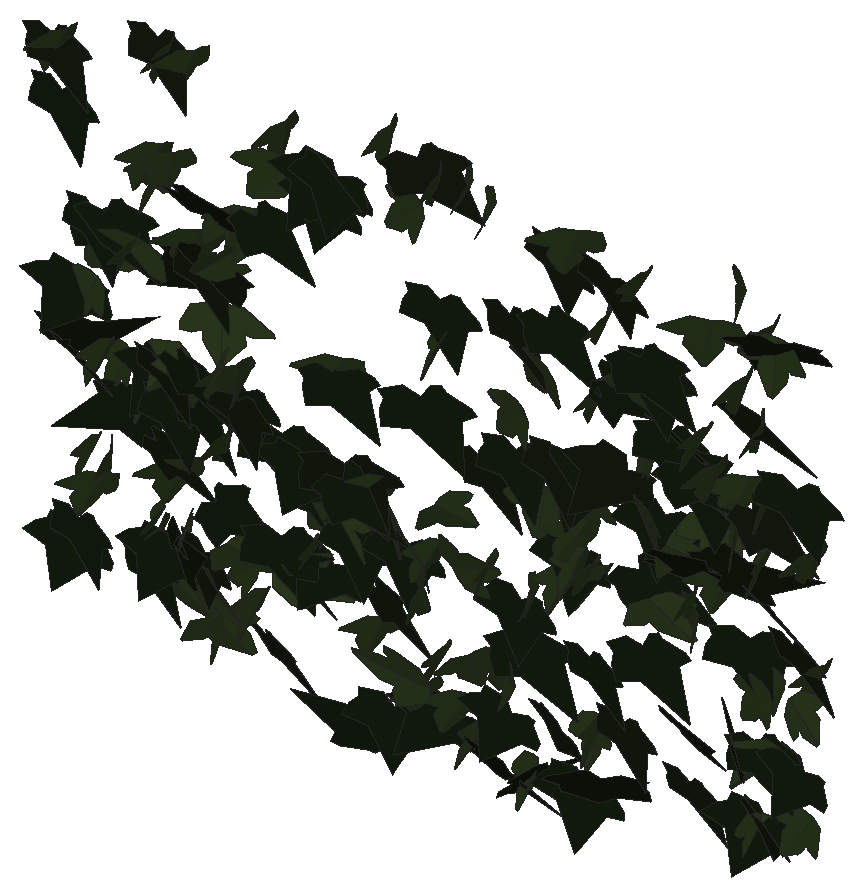
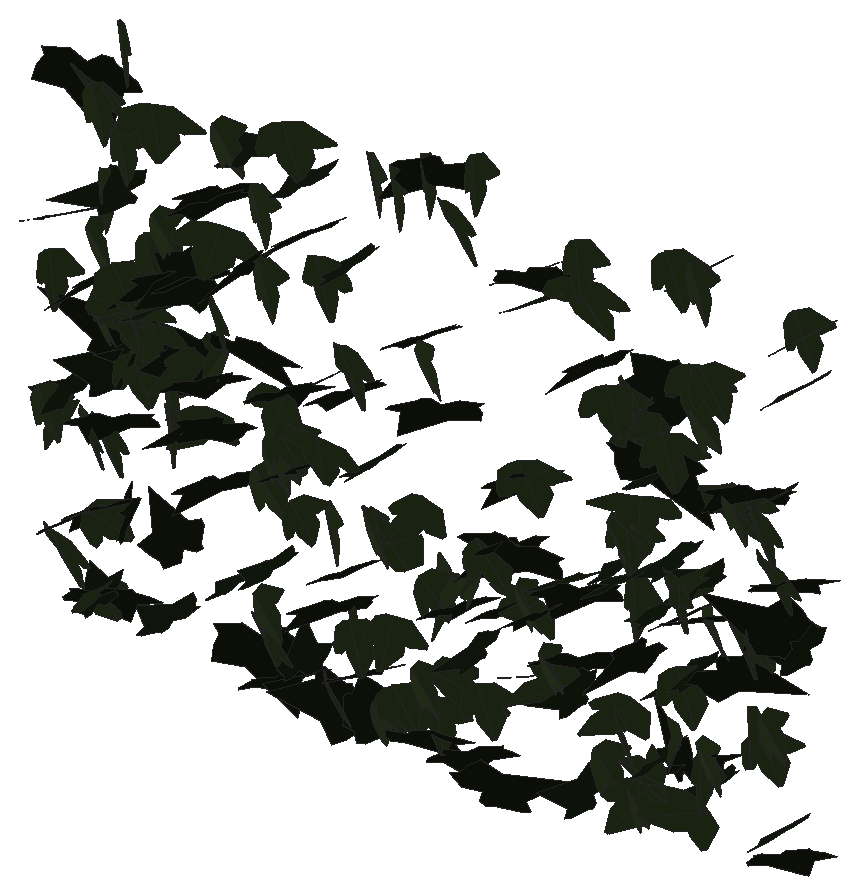
# SketchUp Ruby script. Lengths in millimetres.
U = 1.mm
M = Sketchup.active_model
def pt(a) = Geom::Point3d.new(a.map { |v| v * U })
def face(e, loops, mat)
  f = e.add_face(loops[0].map { |a| pt(a) })
  loops[1..].each { |l| e.add_face(l.map { |a| pt(a) }).erase! }
  f.material = f.back_material = mat if mat
  f
end
# faces: each face lists its corners as indices into pts; further lists are holes
def faces(e, pts, list, mat = nil) = list.each { |f| face(e, (f[0].is_a?(Array) ? f : [f]).map { |l| l.map { |i| pts[i] } }, mat) }
# xy, xz, yz: faces in a plane at the given z, y or x. An outline is a flat list of corners, or four numbers for a rectangle; further outlines are holes
def ring(l) = l.size == 4 ? [[l[0], l[1]], [l[2], l[1]], [l[2], l[3]], [l[0], l[3]]] : l.each_slice(2).to_a
def flat(e, list, mat, &to3) = list.each { |f| face(e, (f[0].is_a?(Array) ? f : [f]).map { |l| ring(l).map { |u, v| to3.(u, v) } }, mat) }
def xy(e, z, list, mat = nil) = flat(e, list, mat) { |x, y| [x, y, z] }
def xz(e, y, list, mat = nil) = flat(e, list, mat) { |x, z| [x, y, z] }
def yz(e, x, list, mat = nil) = flat(e, list, mat) { |y, z| [x, y, z] }
def lines(e, pts, list) = list.each { |a, b| e.add_line(pt(pts[a]), pt(pts[b])) }
# prism: a flat outline (further loops are holes) pulled along v
def prism(e, loops, v, mat = nil)
  f = face(e, loops, mat); d = Geom::Vector3d.new(v.map { |x| x * U })
  f.pushpull(f.normal.samedirection?(d) ? d.length : -d.length)
end
def box(e, o, s, mat = nil) = prism(e, [[o, [o[0] + s[0], o[1], o[2]], [o[0] + s[0], o[1] + s[1], o[2]], [o[0], o[1] + s[1], o[2]]]], [0, 0, s[2]], mat)
def at(x, y, z, deg = 0) = Geom::Transformation.translation(pt([x, y, z])) * Geom::Transformation.rotation(ORIGIN, Z_AXIS, deg.degrees)
def axes(o, x, y, z) = Geom::Transformation.new([*x, 0, *y, 0, *z, 0, *pt(o).to_a, 1])
def part(name) = M.definitions.add(name)
# library, detail: a bought-in or finely detailed component or shape, given as its bounding box
def library(name, o, s) = part(name).tap { |d| box(d.entities, o, s) }
def detail(e, o, s) = box(e.add_group.entities, o, s)
def put(e, d, t, mat = nil) = e.add_instance(d, t).tap { |i| i.material = mat if mat }
def group(e, t, mat = nil) = e.add_group.tap { |g| g.transformation = t; g.material = mat if mat }.entities
root = M.entities
M.materials.add("efeu1").color = [18, 25, 13]
M.materials.add("efeu2").color = [43, 57, 29]
c1 = part("ivyleaf_9")
p = [[39.1,54.8,31.7],[34.5,51.8,30.2],[-5.3,25.2,17.3],[-17.9,28.3,20.9],[-21.6,21.7,17],[-20.2,4.3,5.3],
  [-22.9,-0.3,2.5],[-17.1,-4,-0.6],[-2,-2.1,-1.2],[-0.7,-15.4,-10.1],[16.6,-22.3,-16.7],[21.1,-15.1,-12.5],
  [32.7,-10.7,-11],[46.1,-1.8,-6.6],[30.8,11.2,3.8]]
faces(c1.entities,p,[[0,1,2,3,4,5,6,7,8,9,10,11,12,13,14]],"efeu1")
c2 = part("ivyleaf_10")
p = [[0,12.8,-0.8],[-1.5,51.3,-10.9],[-4.9,51,-11.6],[-13.6,26.5,-7.3],[-13.2,15.9,-4.6],[-21.1,19.3,-7.2],
  [-29.5,16.3,-8.3],[-29.2,8.3,-6.2],[-19.7,-9.8,0.5],[-7.6,-13,4],[1,-12.2,5.8],[-0.4,51.1,-11.1],
  [-1.5,51.1,-10.9],[1,-12.4,5.9],[16.9,-12.4,3.5],[35.1,9.1,-5.1],[35,12.9,-6.1],[20.5,16.4,-4.9],
  [15.8,15,-3.8],[15.3,27.6,-7.1],[12.8,31.3,-7.8]]
faces(c2.entities,p,[[0,1,2,3,4,5,6,7,8,9,10],[11,12,0,13,14,15,16,17,18,19,20]],"efeu2")
put(root,c1,axes([2801.1,826.6,2664.1],[-1.10955,-0.82912,0.08509],[-0.11702,-0.06078,-1.01345],[1.58194,-0.58603,-0.01529]))
put(root,c2,axes([2807.7,780.4,3394.3],[-0.3467,-1.12207,0.06098],[-0.01451,-0.06054,-1.13675],[2.13862,-0.18231,0.00218]))
put(root,c1,axes([2775.7,808.9,2958],[1.15219,-0.84979,0.25487],[0.27577,-0.2097,-1.04338],[1.66582,0.62248,-0.00356]))
put(root,c1,axes([2816.9,808,3034.7],[-1.24222,-0.80833,0.30515],[-0.17317,-0.316,-1.0317],[1.63524,-0.64752,0.12255]))
put(root,c1,axes([2794,785.9,3384.4],[0.30526,-1.10682,-0.1239],[-0.02359,0.1234,-1.11837],[2.11953,0.16078,0.0054]))
put(root,c1,axes([2803.6,791.1,3306.8],[0.05728,-1.13304,0.14401],[-0.01395,-0.14425,-1.13339],[2.1737,0.02893,-0.01107]))
put(root,c1,axes([2806.6,820.6,2691.5],[0.14849,-1.05092,0.15369],[-0.03699,-0.15549,-1.05337],[2.02105,0.07437,-0.03057]))
put(root,c2,axes([2836.9,800.2,3044.7],[1.54076,-0.74256,-0.07024],[-0.09909,0.04716,-1.09854],[1.41609,0.81123,-0.00044]))
put(root,c2,axes([2840.7,803.3,2821.8],[0.26864,-1.00933,0.37026],[0.19743,-0.35891,-1.01793],[2.03658,0.16793,0.04984]))
put(root,c1,axes([2812,803,2958],[0.25424,-0.24109,1.08514],[2.02552,0.34325,-0.05475],[-0.61074,1.03805,0.27013]))
put(root,c2,axes([2849,811.8,3116.8],[1.37351,-0.76625,-0.26758],[-0.18364,0.27452,-1.04638],[1.53374,0.71907,0.11434]))
put(root,c2,axes([2848.9,815.4,2954.1],[-0.04483,-1.01285,0.35435],[0.15288,-0.3551,-1.00967],[2.03649,0.00436,0.08359]))
put(root,c2,axes([2861.5,786.7,2782.8],[-0.75736,-0.95193,0.27209],[-0.06897,-0.27905,-1.02926],[1.88301,-0.3931,0.07174]))
put(root,c1,axes([2843.6,807.7,3140.8],[0.01858,-1.10197,0.19045],[0.00835,-0.19042,-1.10201],[2.12835,0.01036,0.00266]))
put(root,c2,axes([2870.9,797,2819.4],[0.28302,-0.96486,-0.42015],[0.12334,0.43191,-0.96894],[1.99907,0.10995,0.11927]))
put(root,c2,axes([2874.8,818.4,2947.8],[1.28393,-0.84668,-0.05431],[-0.05125,0.04798,-1.08254],[1.6139,0.6751,0.00883]))
put(root,c1,axes([2900.1,820.3,2888.5],[-0.06741,-0.21643,-1.12372],[-0.26118,-1.11534,0.21915],[-2.16226,0.14147,0.00856]))
put(root,c1,axes([2862.3,805.3,3149],[-0.06879,-0.87646,-0.66877],[0.48857,0.64404,-0.85793],[2.04053,-0.18375,0.18287]))
put(root,c2,axes([2907.8,797.3,3122.4],[1.76347,0.1574,-0.59669],[-1.17438,0.22347,-0.89926],[-0.01402,1.07919,0.27324]))
put(root,c2,axes([2900.4,802.6,3121.8],[0.24739,-1.08128,0.03849],[-0.02294,-0.04022,-1.08894],[2.05907,0.12946,-0.01675]))
put(root,c2,axes([2925.9,808.6,2936],[1.02094,-0.86378,0.36948],[0.3238,-0.32912,-1.01643],[1.75847,0.5621,-0.02735]))
put(root,c2,axes([2937.8,807.8,2752.4],[0.47727,-1.00004,0.05704],[-0.01289,-0.06049,-1.03078],[1.90632,0.24996,-0.02125]))
put(root,c2,axes([2936.1,819,3229.4],[0.33367,-0.94598,0.53413],[0.22354,-0.52136,-0.96192],[2.05542,0.21027,0.01791]))
put(root,c2,axes([2941.3,805.3,2732.3],[-0.08638,-0.98582,-0.46393],[0.13683,0.46061,-0.9858],[2.06906,-0.07162,0.04582]))
put(root,c2,axes([2945.3,793.7,3273.5],[-0.45942,-1.07051,0.30346],[-0.00104,-0.31041,-1.09545],[2.11768,-0.2324,0.0653]))
put(root,c1,axes([2945.8,825.3,2946.2],[-1.22139,-0.75796,0.41022],[-0.15538,-0.4557,-0.9697],[1.63289,-0.61031,0.21457]))
put(root,c2,axes([2956.4,800.5,3417.3],[0.14916,-1.1181,-0.11985],[0.03099,0.12126,-1.12057],[2.13993,0.07618,0.02458]))
put(root,c1,axes([2936.6,792,2697.5],[0.47251,-1.02616,0.13462],[0.05397,-0.13165,-1.05576],[1.96897,0.24986,-0.00337]))
put(root,c2,axes([2967.1,794.3,3269.1],[-0.98097,-1.00778,-0.09552],[0.0936,0.08214,-1.13192],[1.92432,-0.51773,0.00636]))
put(root,c1,axes([2948.2,799.4,3427.7],[0.1969,-1.12618,-0.01265],[-0.00764,0.01234,-1.13092],[2.14346,0.1035,-0.00287]))
put(root,c2,axes([2968.2,812.2,2978],[-0.49162,-0.3332,1.00297],[0.29915,-1.03312,-0.30273],[1.98906,0.07303,0.29343]))
put(root,c1,axes([2970.3,792.8,2720.7],[-0.95462,-0.87184,0.30464],[-0.26067,-0.27262,-1.00569],[1.73823,-0.51969,0.01649]))
put(root,c2,axes([2979.8,799.7,2837.4],[-0.88497,-1.06092,0.0823],[-0.029,-0.08316,-1.15818],[2.025,-0.46483,0.01938]))
put(root,c1,axes([2951.6,797.1,2860.4],[1.22153,-0.75905,-0.41264],[-0.26761,0.41541,-0.98287],[1.62236,0.64004,0.14856]))
put(root,c2,axes([2950.3,815.2,2668.4],[-1.41336,0.26915,-0.83997],[1.51063,-0.27496,-0.78985],[-0.73213,-1.08694,-0.00819]))
put(root,c2,axes([2993.8,793.4,2742.7],[0.10618,-0.03913,1.05907],[-0.9757,0.9272,0.06126],[-1.76531,-0.51482,0.02984]))
put(root,c1,axes([2959.6,793.7,2972.2],[0.18973,-0.9481,0.51024],[0.33745,-0.49097,-0.94694],[2.02117,0.17097,0.1102]))
put(root,c2,axes([2992.5,802.7,2972.6],[1.16461,-0.80627,-0.41024],[-0.25459,0.40919,-1.00374],[1.70278,0.61263,0.13051]))
put(root,c2,axes([2995.5,800.6,3421.7],[-0.60731,-1.08053,0.06525],[-0.01505,-0.0657,-1.12661],[2.06015,-0.31901,0.01101]))
put(root,c2,axes([2997.4,808.2,3166.3],[-0.98211,-0.96649,0.0334],[-0.0227,-0.0315,-1.09562],[1.84039,-0.51615,0.00431]))
put(root,c1,axes([2978.2,793,2928.8],[-0.09021,-1.08135,0.06935],[0.01532,-0.06976,-1.08233],[2.0622,-0.04678,0.01108]))
put(root,c1,axes([3027.8,798.5,3141.1],[0.73257,0.23675,-1.07574],[-1.69913,-0.60038,-0.45158],[-1.22786,0.97207,-0.01691]))
put(root,c1,axes([2984.2,794.1,2711.9],[-0.03752,0.14168,1.08472],[0.32188,-1.07146,0.14302],[2.05694,0.17025,-0.00259]))
put(root,c1,axes([2996,783.1,2996.1],[1.01436,-0.92924,-0.2297],[-0.06113,0.2454,-1.06727],[1.82073,0.52593,0.09214]))
put(root,c1,axes([3008.2,814.4,2716.8],[-0.04258,-0.91012,0.53359],[-0.05345,-0.53301,-0.91031],[2.00719,-0.0335,-0.01292]))
put(root,c1,axes([2999.2,806,2935.1],[0.65484,-1.06382,-0.00474],[-0.00264,0.00453,-1.11808],[2.02468,0.34407,0.00007]))
put(root,c1,axes([3009.8,807.8,3123.6],[0.16596,-1.02644,0.33344],[0.24682,-0.32214,-1.02556],[2.03913,0.12253,0.097]))
put(root,c1,axes([3002.1,783.3,3233.9],[2.01866,-0.29857,0.25163],[0.46138,-0.06743,-1.10189],[0.58255,1.08802,0.00076]))
put(root,c2,axes([3040.1,779,3188.3],[-0.03065,-0.263,-1.09291],[0.38139,1.07484,-0.2616],[2.10514,-0.19856,0.03148]))
put(root,c2,axes([3015.1,803.6,2684.5],[0.2018,-0.24599,1.06458],[1.86659,-0.45001,-0.20167],[0.91657,0.9706,0.1763]))
put(root,c2,axes([3041,804.7,3069],[1.74046,0.73038,-0.01547],[-0.0229,-0.00973,-1.17036],[-1.39019,0.91457,-0.00009]))
put(root,c2,axes([3049.4,803.1,2646.5],[0.40297,-0.93259,0.56746],[0.48337,-0.52009,-0.94951],[2.02064,0.3104,0.11397]))
put(root,c2,axes([3048.8,789.9,2646.8],[-1.28421,-0.71201,-0.63835],[0.87314,0.44445,-0.98068],[1.59683,-0.81563,0.02286]))
put(root,c2,axes([3064.3,760.5,3000.3],[0.61566,-0.58164,0.93153],[-0.68081,0.86234,0.66266],[-1.97612,-0.4783,0.06192]))
put(root,c2,axes([3051.7,774.7,3153.4],[-0.23507,-0.9066,0.74321],[0.39597,0.7185,0.91105],[-2.1957,0.22663,0.08473]))
put(root,c2,axes([3070.8,774.3,2923.9],[-0.12163,-1.06831,-0.50269],[0.08116,0.50101,-1.07016],[2.24559,-0.07597,0.01145]))
put(root,c2,axes([3076.5,821.2,3214.2],[-1.30011,-0.83444,0.20316],[0.07192,-0.28855,-1.05808],[1.63292,-0.65166,0.20836]))
put(root,c2,axes([3076.1,789.5,3208.9],[0.89561,-0.88521,-0.483],[-0.17837,0.4923,-0.99357],[1.9109,0.46084,0.13363]))
put(root,c2,axes([3076.4,785.9,3014.6],[-0.62048,-1.04852,-0.2068],[0.07271,0.20464,-1.09778],[2.03269,-0.32738,-0.02386]))
put(root,c1,axes([3063.1,828,2957],[-0.15055,-1.0106,0.33071],[0.09437,-0.33477,-1.01114],[2.02153,-0.05963,0.07183]))
put(root,c1,axes([3071.6,763.1,2832.9],[0.56478,-0.38248,-1.01683],[-0.57943,0.98256,-0.45844],[1.98475,0.39569,0.15551]))
put(root,c2,axes([3086.4,796.8,3009.6],[0.68089,-0.99235,0.27961],[0.18668,-0.26186,-1.05486],[1.95328,0.37095,0.00335]))
put(root,c2,axes([3101.5,786,2745.9],[0.74728,-0.81638,-0.65059],[-0.57799,0.5757,-0.90568],[1.90083,0.496,-0.01962]))
put(root,c2,axes([3075.7,791.2,2760.1],[-0.89734,-0.54655,-0.78965],[1.11831,0.53162,-0.7188],[1.44567,-0.75048,0.06589]))
put(root,c2,axes([3096.3,809.5,2689.5],[0.04555,-1.10375,0.38166],[0.18241,-0.37859,-1.1009],[2.21519,0.05387,0.08281]))
put(root,c1,axes([3076.7,796.9,2962.8],[0.06205,-1.04881,0.30759],[0.07786,-0.30634,-1.04889],[2.07872,0.04278,0.0301]))
put(root,c1,axes([3116.1,787.4,3239.4],[0.52479,-0.86201,-0.65588],[-0.12117,0.66273,-0.89778],[2.05791,0.25885,0.1144]))
put(root,c1,axes([3127.4,818.6,2923.1],[-0.50853,-0.92808,-0.50235],[0.28162,0.48014,-0.96574],[1.98863,-0.30532,0.0083]))
put(root,c2,axes([3152,785,3324.8],[2.02019,-0.00633,-0.42592],[-0.79274,0.22396,-1.0414],[0.16969,1.12159,0.20554]))
put(root,c1,axes([3113.9,812,2635.3],[1.05475,-0.86163,0.22518],[0.22232,-0.1926,-1.02445],[1.68028,0.56634,-0.0058]))
put(root,c2,axes([3148.7,791.6,3380],[-0.30628,-1.08433,-0.26183],[0.15649,0.25229,-1.09536],[2.11722,-0.17551,0.04309]))
put(root,c1,axes([3135.1,805.5,2769.8],[1.23589,-0.80947,-0.00179],[-0.00198,0.00145,-1.03776],[1.54059,0.64938,0.0001]))
put(root,c1,axes([3154.5,786,2801.8],[-0.37692,-1.00307,-0.49728],[0.25916,0.47967,-1.02178],[2.11495,-0.23754,0.03658]))
put(root,c1,axes([3176.5,800.9,2905.9],[-0.84814,-0.85693,0.48361],[-0.0134,-0.5281,-0.94227],[1.87266,-0.39189,0.21228]))
put(root,c2,axes([3184.6,808.8,2795.3],[0.52816,-0.93345,0.37983],[0.17185,-0.36935,-0.97367],[1.91027,0.29131,-0.01742]))
put(root,c2,axes([3172.5,784.5,2759.6],[0.43302,0.55169,1.03329],[0.77933,0.94872,-0.59671],[-2.08864,0.46837,-0.00843]))
put(root,c1,axes([3184.8,820.2,2871.7],[0.03766,-1.06474,-0.17642],[0.03095,0.17673,-1.06475],[2.05381,0.01686,0.01928]))
put(root,c2,axes([3216.1,817.5,3055.7],[-1.10488,-0.8867,0.28565],[-0.12945,-0.29533,-1.055],[1.76825,-0.57567,0.10125]))
put(root,c1,axes([3206.7,815,2771.2],[-1.20431,-0.75503,0.33523],[0.05966,-0.44392,-0.94065],[1.57112,-0.5619,0.29269]))
put(root,c1,axes([3221.3,801.1,3329.5],[-1.55457,-0.76542,0.12972],[-0.19788,-0.07874,-1.11932],[1.46421,-0.8233,-0.01355]))
put(root,c1,axes([3208,806.4,3295.2],[-0.67101,-0.96913,0.4354],[0.00732,-0.45991,-1.02057],[2.02203,-0.31994,0.14818]))
put(root,c2,axes([3229,800.7,2867.3],[0.54968,-0.95997,0.405],[0.22514,-0.38734,-1.00247],[1.97013,0.3121,0.00156]))
put(root,c1,axes([3225.6,802.9,3328.8],[-0.62155,-1.01037,0.36855],[0.00722,-0.38624,-1.05553],[2.04686,-0.30545,0.11563]))
put(root,c1,axes([3217,809.4,3046],[0.09627,-0.93908,-0.57946],[0.08143,0.5813,-0.93833],[2.09854,0.02052,0.063]))
put(root,c2,axes([3222.5,795,2857.6],[-1.5579,0.17952,-0.63499],[0.94862,-0.49483,-0.78243],[-0.82302,-0.91017,0.30014]))
put(root,c1,axes([3292.4,796.3,2570.5],[-0.05748,0.01725,1.01443],[-1.929,0.04513,-0.03094],[-0.08684,-1.01388,0.01588]))
put(root,c1,axes([3244.4,797,2931.3],[-0.88501,-0.58652,-0.85049],[1.03737,0.65302,-0.74836],[1.6703,-0.71633,0.01415]))
put(root,c2,axes([3281.8,816.6,2716.7],[-0.74978,-0.96695,0.11113],[-0.03449,-0.11258,-1.04381],[1.85209,-0.39355,0.02555]))
put(root,c2,axes([3285.2,808.6,2917.7],[-0.63795,-0.97831,0.34484],[-0.13628,-0.33971,-1.03336],[1.96949,-0.3404,0.04019]))
put(root,c1,axes([3264.7,798.5,2839.8],[-0.32243,-1.05432,0.10786],[-0.03368,-0.1064,-1.06784],[2.01677,-0.17034,-0.00059]))
put(root,c1,axes([3259.9,778.5,2923.1],[0.54026,-0.80489,-0.85135],[-0.20004,0.85495,-0.84334],[2.22079,0.27282,0.13114]))
put(root,c2,axes([3295.7,815.8,2880.4],[-0.73097,0.87166,-0.47073],[0.27309,-0.4506,-0.95146],[-1.86552,-0.40751,0.04517]))
put(root,c1,axes([3295,800.4,2770.9],[1.1211,-0.86857,-0.22769],[-0.19,0.20727,-1.04896],[1.69832,0.59655,0.03295]))
put(root,c2,axes([3319.6,783.7,3437.3],[0.02878,-1.1208,-0.20504],[0.2265,0.20549,-1.11448],[2.15664,-0.00662,0.11978]))
put(root,c1,axes([3319.3,797.6,2616],[-0.8006,-0.93913,-0.16507],[0.09988,0.15734,-1.02891],[1.812,-0.42361,-0.01622]))
put(root,c1,axes([3319.6,825.1,2833.8],[-0.4963,-1.0379,0.06941],[-0.00385,-0.07105,-1.07005],[1.97975,-0.26033,0.01532]))
put(root,c2,axes([3371.8,766.9,2687.9],[0.20057,-0.0531,-1.15192],[-1.86778,0.60323,-0.11759],[1.15235,0.98698,0.0099]))
put(root,c2,axes([3367.3,771.6,3351.6],[1.1927,-0.76033,-0.53499],[-0.59418,0.4356,-0.98479],[1.66662,0.69942,0.03176]))
put(root,c2,axes([3361.7,823,2847.1],[-0.20233,-0.96679,0.45959],[0.09431,-0.4658,-0.96839],[2.03513,-0.07453,0.09057]))
put(root,c2,axes([3364.3,800.5,2661.5],[-0.55639,-0.9761,-0.13873],[0.03813,0.13879,-1.01873],[1.87599,-0.29232,-0.02044]))
put(root,c2,axes([3348.6,808.8,2829.4],[-1.08645,0.30448,0.89081],[1.12243,-0.69636,0.61595],[1.39653,0.79656,0.19796]))
put(root,c2,axes([3377.7,819.7,2707.9],[0.30382,-1.00517,0.26184],[0.06061,-0.26005,-1.01772],[1.97594,0.16253,-0.00904]))
put(root,c2,axes([3375,775.2,2810.7],[0.30188,-0.89196,-0.66582],[0.2691,0.68325,-0.88162],[2.10123,0.04064,0.20856]))
put(root,c1,axes([3390.2,817.4,2624.5],[-1.63004,-0.54311,0.17545],[-0.21037,-0.15257,-1.01183],[1.06568,-0.86085,0.06863]))
put(root,c2,axes([3382.2,807.5,3153.2],[0.73159,-0.99544,0.22732],[0.13009,-0.21726,-1.06698],[1.93893,0.39017,-0.01418]))
put(root,c1,axes([3373.7,821.7,3197],[-0.22637,-1.08675,-0.01996],[0.12549,0.01283,-1.09136],[2.06484,-0.11992,0.06414]))
put(root,c1,axes([3377.3,781.4,3079.2],[-0.36108,-0.94602,-0.63753],[0.4203,0.60361,-0.9614],[2.13008,-0.27946,0.08163]))
put(root,c1,axes([3376.3,778.5,3417],[0.01715,-0.68641,-0.91145],[0.32487,0.90203,-0.67763],[2.14713,-0.131,0.10981]))
put(root,c2,axes([3402.9,775.5,3404.7],[0.30135,-1.07209,-0.37597],[0.05877,0.38352,-1.08062],[2.16143,0.13904,0.0818]))
put(root,c2,axes([3397.9,793.8,2930.3],[-0.78009,-0.64076,-0.76736],[0.79321,0.64432,-0.76064],[1.72942,-0.58455,0.00274]))
put(root,c2,axes([3421.6,805.9,2661.7],[-0.89892,-0.87369,0.2882],[-0.19876,-0.27095,-0.99255],[1.73962,-0.48242,0.03552]))
put(root,c2,axes([3427.5,806.2,3390.9],[0.37874,-1.02755,-0.40769],[-0.00954,0.4134,-1.04439],[2.10392,0.18685,0.06866]))
put(root,c2,axes([3449.8,804.8,2629.9],[0.19351,-0.89329,0.61369],[0.16747,-0.60755,-0.89893],[2.05585,0.13357,0.01546]))
put(root,c2,axes([3451.5,782.5,2739.3],[-0.89602,-0.85884,-0.41169],[0.31756,0.37776,-0.97887],[1.7846,-0.49843,-0.03252]))
put(root,c2,axes([3427.3,793.3,2853.6],[-1.28439,0.17521,0.84981],[1.58218,-0.1778,0.69684],[0.47299,1.07051,-0.02335]))
put(root,c1,axes([3440.8,822.7,2996.8],[0.5155,-1.05188,-0.0887],[-0.02406,0.08833,-1.08615],[2.0089,0.27098,0.00975]))
put(root,c2,axes([3479,786.1,3385.3],[0.44018,-0.97472,-0.53381],[-0.15582,0.52882,-1.00109],[2.10932,0.24247,0.03744]))
put(root,c2,axes([3476.2,791,2879.2],[0.43413,-1.02347,0.10611],[0.05246,-0.10257,-1.04857],[1.9576,0.22972,0.00457]))
put(root,c2,axes([3485.1,815.8,2736],[-0.61592,-1.00449,-0.06189],[-0.00211,0.06537,-1.05512],[1.91536,-0.32294,-0.02106]))
put(root,c1,axes([3495.5,805.2,2666.8],[-0.95765,-0.81706,0.39442],[-0.13276,-0.41484,-0.94836],[1.72162,-0.48648,0.14626]))
put(root,c2,axes([3516.4,778.1,2730.7],[0.18166,-0.52779,-0.96309],[-0.41697,0.93814,-0.53583],[2.04814,0.2378,-0.02367]))
put(root,c2,axes([3513.2,793.4,3104.2],[1.35276,-0.66199,-0.52453],[-0.41002,0.52077,-0.94919],[1.55428,0.71354,0.20613]))
put(root,c1,axes([3467.4,785,2609.8],[1.47535,-0.5989,0.50781],[0.7586,-0.31467,-0.97959],[1.28755,0.87165,-0.00473]))
put(root,c1,axes([3498.7,821.8,2819.6],[-0.45755,-1.04013,0.19968],[-0.01686,-0.20277,-1.06694],[2.01566,-0.23781,0.0364]))
put(root,c1,axes([3508.1,792.3,3237],[0.5053,-1.08538,0.06413],[0.02031,-0.06341,-1.11737],[2.06919,0.26567,-0.00469]))
put(root,c1,axes([3520,788.2,3052.2],[-0.21479,-1.0882,-0.13553],[0.04821,0.13362,-1.09398],[2.0865,-0.11511,0.01133]))
put(root,c1,axes([3511.6,815.8,2767.3],[0.16367,-1.05613,-0.5701],[0.21837,0.57618,-1.05009],[2.27372,0.02069,0.14189]))
put(root,c2,axes([3546.4,786.4,2866.8],[0.50144,-0.99616,-0.40747],[-0.07185,0.41069,-1.02844],[2.04711,0.25842,0.06371]))
put(root,c2,axes([3536.1,817.6,2982.3],[2.0048,-0.18903,0.03298],[0.09768,0.10023,-1.06478],[0.35188,1.04912,0.10766]))
put(root,c2,axes([3543.2,785.8,2617.5],[1.13114,-0.90486,0.25286],[0.28287,-0.20489,-1.08253],[1.76559,0.61253,0.01143]))
put(root,c1,axes([3534.4,773.4,2599.2],[-0.01011,0.96764,-0.6836],[-0.17697,0.68116,0.96491],[2.24787,0.05798,0.07289]))
put(root,c2,axes([3567,824.9,2881.9],[-0.33826,-0.95896,0.42217],[0.21639,-0.44332,-0.95914],[1.98235,-0.11524,0.17674]))
put(root,c2,axes([3573.3,767.2,3196.6],[1.52124,-0.48239,-0.64322],[-0.38556,0.75689,-0.81939],[1.48081,0.69263,0.44743]))
put(root,c1,axes([3565.6,820.1,2659.7],[-0.5343,-0.40803,0.92483],[0.18253,-0.96626,-0.39719],[1.91515,-0.02174,0.29587]))
put(root,c1,axes([3569,812.1,3047.8],[-0.11608,-1.09203,0.20003],[-0.01998,-0.19976,-1.09373],[2.11284,-0.06188,0.00065]))
put(root,c1,axes([3571.8,811.7,3336.4],[-0.19272,-0.97599,0.52165],[0.13105,-0.52837,-0.9752],[2.1021,-0.05654,0.10862]))
put(root,c2,axes([3604,808.9,2967.1],[-0.54507,-0.94984,0.42976],[-0.04052,-0.44026,-0.98724],[1.98375,-0.26998,0.09792]))
put(root,c1,axes([3576.7,783.1,3258.3],[0.48974,-1.02174,-0.43615],[0.01394,0.44925,-1.0481],[2.11429,0.2337,0.10794]))
put(root,c2,axes([3610.6,791.8,3385.1],[-1.22742,-0.93034,0.15816],[-0.08308,-0.16194,-1.13064],[1.7941,-0.64398,0.05584]))
put(root,c1,axes([3598.2,819.9,3037.9],[-0.87758,-0.97307,0.1304],[-0.08183,-0.12391,-1.07671],[1.86671,-0.4629,0.0141]))
put(root,c1,axes([3593.6,814.3,2923.4],[-0.52797,-1.00563,0.23315],[-0.07418,-0.23105,-1.04294],[1.96329,-0.27917,0.02329]))
put(root,c2,axes([3608.7,810.5,3016.3],[-1.74567,0.56518,0.07249],[-0.18468,-0.01957,-1.07526],[-1.06862,-0.91988,0.06741]))
put(root,c2,axes([3611.4,800.4,2944.6],[0.25544,-1.0736,0.58604],[0.39138,-0.56136,-1.07548],[2.29473,0.21525,0.11819]))
put(root,c2,axes([3613.9,789.1,2937.6],[-0.09213,-0.89408,0.60434],[0.38402,-0.60178,-0.87413],[2.01766,0.07371,0.19397]))
put(root,c2,axes([3624.9,820.1,2905.1],[-0.06587,-1.04937,0.32883],[-0.04598,-0.32818,-1.04986],[2.09241,-0.04025,-0.01272]))
put(root,c2,axes([3618.6,820.1,2687.1],[1.48048,-0.67667,0.3183],[0.40595,-0.23943,-1.03029],[1.36408,0.80567,-0.03884]))
put(root,c1,axes([3622.5,795,2615.5],[-0.73986,-1.06838,0.09552],[-0.06624,-0.08898,-1.13691],[2.04038,-0.39029,-0.00227]))
put(root,c2,axes([3633.7,791.5,2927.7],[0.20998,-1.05731,0.12968],[0.00023,-0.13036,-1.06297],[2.02735,0.10952,-0.01331]))
put(root,c1,axes([3614.2,816.5,2779.7],[0.45368,-1.02478,0.17504],[0.10984,-0.16626,-1.05198],[1.97556,0.24458,0.01829]))
put(root,c2,axes([3641.7,798,3179.8],[0.08131,-1.1123,-0.13027],[0.04062,0.13115,-1.11281],[2.13101,0.03994,0.02618]))
put(root,c2,axes([3643.5,798.1,2710.5],[0.37846,-1.10467,0.40504],[0.24123,-0.38828,-1.12119],[2.22624,0.22987,0.05263]))
put(root,c2,axes([3649.7,800.4,3284.8],[0.14483,-1.0816,-0.29426],[-0.06062,0.29273,-1.08422],[2.13246,0.08178,-0.01084]))
put(root,c1,axes([3662.5,775.1,2645.8],[0.72824,0.88653,-0.68701],[-0.6185,-0.60711,-0.96444],[-2.043,0.49981,0.04708]))
put(root,c1,axes([3675.3,806.7,3072.5],[-2.00682,-0.26332,-0.06963],[0.12162,0.03147,-1.08672],[0.50391,-1.05627,-0.01501]))
put(root,c1,axes([3655.4,795.8,3196.2],[0.89342,-0.40472,-0.9178],[-0.7195,0.86722,-0.57578],[1.76826,0.55736,0.22944]))
put(root,c1,axes([3662.7,796.6,3341.2],[-0.05559,-0.96271,0.57528],[0.34988,-0.5718,-0.94756],[2.10557,0.0696,0.17264]))
put(root,c2,axes([3704.6,803.5,3356.5],[0.18607,-1.07825,0.26087],[-0.01955,-0.26275,-1.08217],[2.11125,0.09259,-0.03301]))
put(root,c1,axes([3686.7,791.3,2724.4],[0.17918,-1.01917,0.23102],[0.08335,-0.22791,-1.02327],[1.98714,0.10146,0.02209]))
put(root,c2,axes([3710,812.1,3116.1],[1.02892,-0.95786,-0.16865],[-0.01125,0.18972,-1.09644],[1.85101,0.5336,0.08709]))
put(root,c2,axes([3710.9,805,3212.3],[-1.86623,-0.49484,-0.17897],[0.28551,0.0999,-1.09815],[0.95992,-0.99176,-0.02132]))
put(root,c2,axes([3717.7,789.5,3041.2],[-1.02995,0.92083,-0.21138],[0.16513,-0.19413,-1.06783],[-1.7905,-0.54759,0.02311]))
put(root,c1,axes([3719.9,829,3013.8],[-0.77013,-1.00898,0.01705],[0.01295,-0.02109,-1.087],[1.92052,-0.40446,0.01416]))
put(root,c1,axes([3709.1,799.9,2943.9],[0.49069,-0.61874,-0.88905],[0.32266,0.92568,-0.59506],[2.03607,0.00242,0.30856]))
put(root,c1,axes([3727.1,781.8,2850.5],[0.15388,-1.00803,-0.59661],[-0.02583,0.59719,-1.01084],[2.22918,0.07651,0.02947]))
put(root,c1,axes([3734.7,791.6,3246.9],[-0.30513,-1.12703,-0.08932],[0.00131,0.09012,-1.13832],[2.1517,-0.15988,-0.01198]))
put(root,c1,axes([3727.9,777.1,3259.2],[0.2046,-0.93748,-0.60834],[0.18217,0.61663,-0.93334],[2.11914,0.0375,0.13897]))
put(root,c1,axes([3743.5,809.4,3143.2],[-0.07259,-1.08994,-0.24088],[0.00228,0.24098,-1.09058],[2.12443,-0.0375,-0.00706]))
put(root,c1,axes([3738.2,810.9,3148.6],[1.94836,-0.3629,-0.18858],[-0.32849,0.07747,-1.08604],[0.70565,1.03807,0.01512]))
put(root,c2,axes([3752.8,772.6,2924.4],[-1.11317,-0.70495,-0.56787],[1.03721,0.26561,-0.89106],[1.37562,-0.77073,0.21233]))
put(root,c2,axes([3769.4,784.7,3006.1],[-0.35295,-0.69008,-0.87003],[0.92748,0.74203,-0.69243],[1.89908,-0.49065,0.17647]))
put(root,c2,axes([3797.1,787.7,2918.4],[0.78608,-0.76351,-0.7131],[-0.18097,0.73616,-0.84327],[1.98008,0.37039,0.20603]))
put(root,c1,axes([3768.6,821.4,2656.3],[0.34317,-0.95699,0.36294],[0.38872,-0.32748,-0.96494],[1.90875,0.23875,0.13126]))
put(root,c2,axes([3805.1,777.5,2959.5],[0.22407,-1.03486,-0.41635],[0.07169,0.42211,-1.03853],[2.12175,0.09503,0.07906]))
put(root,c1,axes([3773.9,795.6,2746.9],[1.57984,-0.32,-0.56805],[1.02024,-0.18847,0.88952],[-0.70628,-0.98804,0.0143]))
put(root,c1,axes([3784.3,795.1,3120.7],[0.4304,-0.63801,-0.89851],[0.11389,0.92299,-0.64034],[2.09421,0.08093,0.21948]))
put(root,c1,axes([3768.6,770.3,2994.1],[1.6157,-0.0895,0.67242],[1.29078,0.13362,-0.83847],[-0.02594,1.07471,0.16025]))
put(root,c2,axes([3813.9,786.7,3182.9],[0.27149,-1.05802,0.31881],[0.02619,-0.31973,-1.06723],[2.1029,0.14057,-0.02787]))
put(root,c1,axes([3799.1,816,3081.7],[-0.31281,-1.00943,0.40946],[0.20948,-0.42737,-1.00939],[2.06258,-0.10968,0.16461]))
put(root,c2,axes([3824.4,789,3334.4],[-1.59092,-0.75041,0.11104],[-0.02163,-0.15283,-1.11835],[1.44356,-0.8293,0.10562]))
put(root,c2,axes([3836.1,780.3,3142.6],[-0.24653,-1.12733,-0.11178],[0.04309,0.10991,-1.1347],[2.15562,-0.13113,0.0099]))
put(root,c2,axes([3839.8,802.5,2984],[-0.8496,-0.98521,0.21774],[-0.01454,-0.2348,-1.07802],[1.92024,-0.43768,0.08817]))
put(root,c2,axes([3823.4,807.3,3044.4],[1.99713,0.34469,0.06041],[0.11759,0.00547,-1.10443],[-0.65556,1.05108,-0.01407]))
put(root,c2,axes([3852.1,811.1,3072.8],[-1.94427,-0.29347,0.28723],[-0.48905,-0.14386,-1.06091],[0.60961,-1.0514,0.06499]))
put(root,c2,axes([3855.5,818.6,3111.8],[-0.94032,-0.95007,0.25956],[0.01813,-0.29498,-1.06161],[1.87435,-0.47378,0.14048]))
put(root,c2,axes([3852.9,802.8,3062.3],[0.85665,-0.89395,0.51532],[0.63212,-0.40677,-0.99575],[1.85929,0.55017,0.10111]))
put(root,c1,axes([3880.6,779.3,2738.1],[-0.14236,-0.53798,0.91294],[0.2395,0.90423,0.54316],[-2.00249,0.14639,0.00006]))
put(root,c2,axes([3881.6,778.6,3282.9],[-0.06396,-1.14125,-0.19402],[0.0898,0.19259,-1.14101],[2.20136,-0.04101,0.04091]))
put(root,c1,axes([3885.3,816.2,2650.3],[-1.4176,-0.7469,-0.04319],[0.05715,0.03105,-1.05483],[1.42274,-0.74545,-0.00066]))
put(root,c2,axes([3889.3,766.4,3417.7],[0.60387,-0.83678,-0.7553],[-0.20908,0.75796,-0.88588],[2.13517,0.31088,0.12687]))
put(root,c2,axes([3887.7,809.1,2647.2],[0.67821,0.86532,-0.42603],[-0.46317,-0.35882,-0.93236],[-1.77627,0.42396,0.08045]))
put(root,c1,axes([3872.1,808.7,2899.5],[-0.5602,-0.98666,-0.40915],[0.35217,0.37088,-1.0275],[2.00213,-0.34131,0.06625]))
put(root,c2,axes([3896.5,808.8,2751.1],[-0.36435,-0.69625,0.81307],[-0.05483,-0.82232,-0.71096],[2.03653,-0.1467,0.12632]))
put(root,c1,axes([3857.4,801.3,3224],[1.47972,-0.80115,-0.05837],[0.2792,0.22148,-1.08589],[1.50307,0.74756,0.25917]))
put(root,c2,axes([3897,811.2,3346.7],[-0.10699,-1.10216,-0.15484],[-0.00899,0.15527,-1.10352],[2.11822,-0.05501,-0.01251]))
put(root,c2,axes([3898.1,791.9,3218],[0.2176,-1.03129,-0.49062],[0.0139,0.49372,-1.03611],[2.17349,0.10009,0.05574]))
put(root,c1,axes([3861.4,813.7,2973.5],[1.16222,-0.84668,0.39602],[0.43578,-0.32313,-1.04392],[1.72476,0.65218,-0.0031]))
put(root,c1,axes([3854.8,781,2999.2],[0.31499,-0.06758,1.13669],[2.0688,-0.33275,-0.17806],[0.6455,1.09942,0.01598]))
put(root,c2,axes([3901.3,796.8,3033.8],[0.6632,-0.95776,0.37295],[0.22752,-0.35336,-1.01915],[1.94286,0.36832,-0.00796]))
put(root,c1,axes([3885.8,821.4,2640.9],[-0.11014,-0.59802,0.85251],[0.17235,-0.85348,-0.59256],[1.97439,0.04114,0.09928]))
put(root,c2,axes([3913.8,773.5,2855.7],[1.31308,-0.7307,-0.37216],[-0.31253,0.35339,-0.99829],[1.52904,0.69973,0.11555]))
put(root,c1,axes([3892.1,800.9,2763.1],[0.02602,-0.99533,-0.36117],[0.07561,0.36142,-0.99454],[2.01375,-0.00071,0.04201]))
put(root,c1,axes([3890.4,794.7,3094.4],[0.83614,-0.82855,-0.72022],[-0.27976,0.72437,-0.92299],[2.07056,0.43246,0.16613]))
put(root,c2,axes([3912.6,793.9,3135.4],[0.63339,-0.94895,0.48305],[0.38342,-0.44084,-1.00482],[1.98996,0.38698,0.03986]))
put(root,c2,axes([3928,789.2,2864.6],[0.98542,-0.93369,-0.10677],[-0.07079,0.10144,-1.06751],[1.78717,0.51884,0.01658]))
put(root,c1,axes([3941.6,772,3359.2],[1.03509,0.81806,-0.55742],[-0.85729,-0.36183,-0.97051],[-1.67766,0.68963,0.15202]))
put(root,c2,axes([3926.5,785.1,3341.8],[1.959,-0.45344,0.24378],[0.43782,-0.08244,-1.12464],[0.87655,1.05458,0.0169]))
put(root,c1,axes([3942.5,821.7,2733.6],[-0.71119,-0.83565,0.61182],[-0.34329,-0.58797,-0.91325],[1.94098,-0.41018,0.06266]))
put(root,c1,axes([3938.4,812.6,2911.8],[0.58883,-0.98509,0.32567],[0.23759,-0.30203,-1.03217],[1.96028,0.33251,0.02728]))
put(root,c2,axes([3969.6,791,2684.8],[1.53672,-0.71475,-0.19769],[-0.27836,0.13303,-1.07835],[1.38367,0.82058,0.00262]))
put(root,c2,axes([3976.9,812.5,2893.7],[-0.11178,-1.07905,0.08087],[0.02362,-0.08166,-1.08052],[2.05928,-0.05764,0.01678]))
put(root,c1,axes([3961,789.2,3150.8],[-0.34875,-1.09774,-0.03723],[0.40383,0.00166,-1.09315],[2.05105,-0.18698,0.2089]))
put(root,c2,axes([3985.6,785,3070.8],[-0.33118,-1.07449,-0.26448],[0.1152,0.25809,-1.08834],[2.10285,-0.18336,0.01797]))
put(root,c2,axes([3977.6,770.1,2858.6],[0.0884,1.0087,0.41836],[-0.13517,0.42065,-1.00632],[-2.07393,0.01558,0.08342]))
